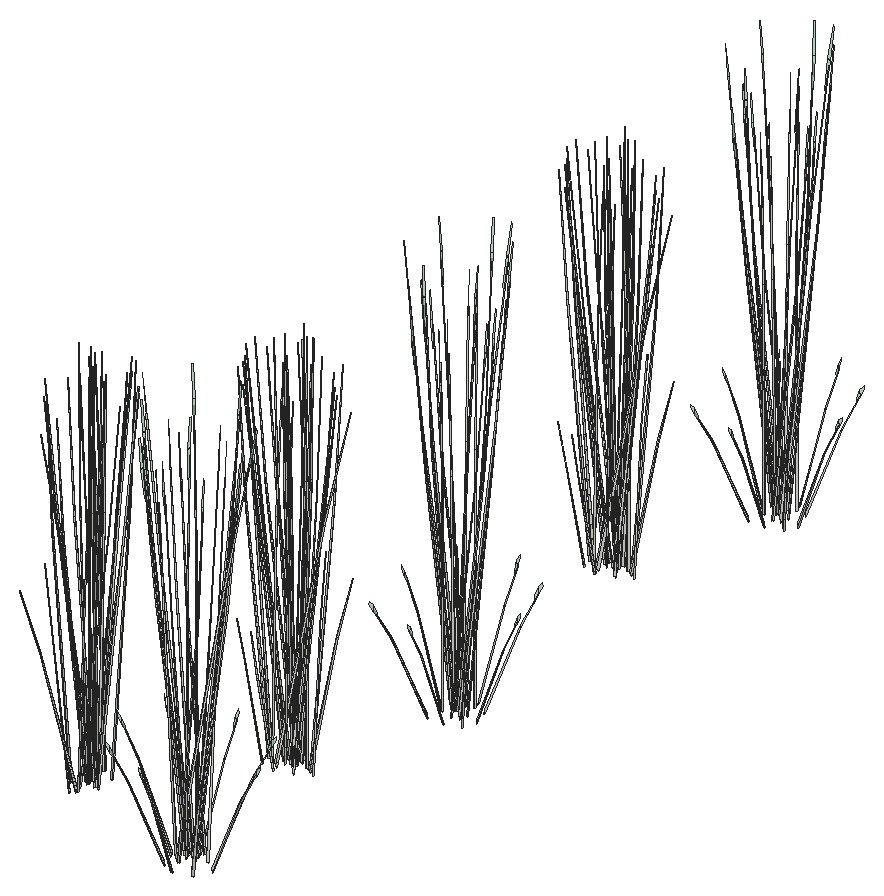
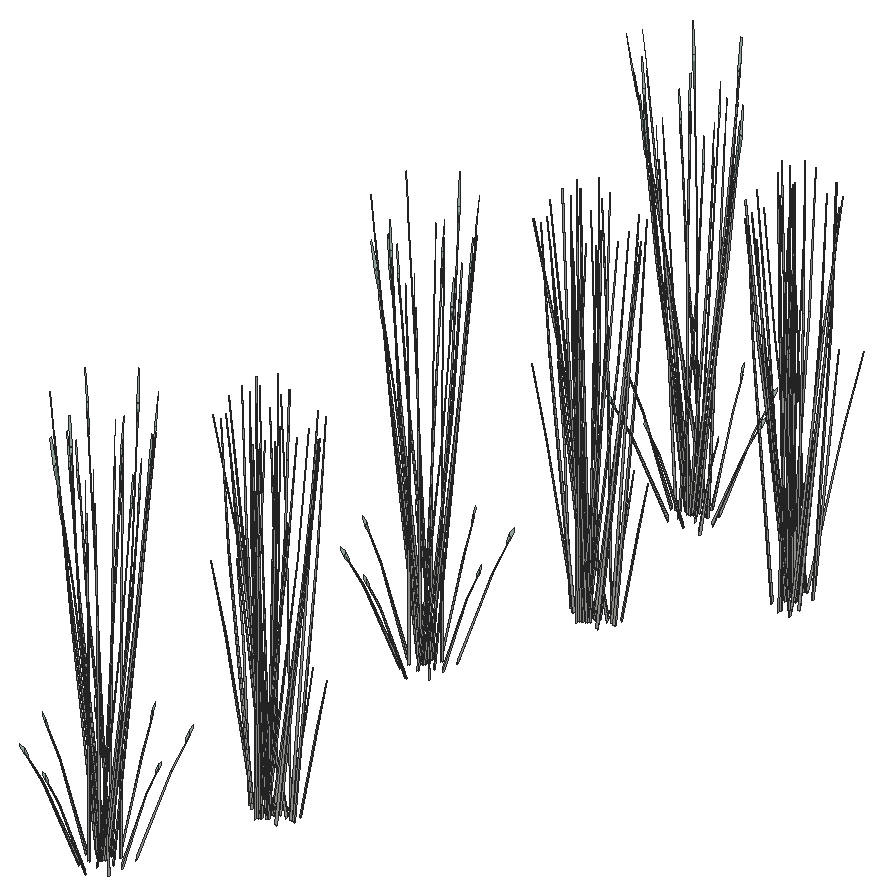
# SketchUp Ruby script. Lengths in inches.
U = 1.inch
M = Sketchup.active_model
def pt(a) = Geom::Point3d.new(a.map { |v| v * U })
def face(e, loops, mat)
  f = e.add_face(loops[0].map { |a| pt(a) })
  loops[1..].each { |l| e.add_face(l.map { |a| pt(a) }).erase! }
  f.material = f.back_material = mat if mat
  f
end
# faces: each face lists its corners as indices into pts; further lists are holes
def faces(e, pts, list, mat = nil) = list.each { |f| face(e, (f[0].is_a?(Array) ? f : [f]).map { |l| l.map { |i| pts[i] } }, mat) }
# xy, xz, yz: faces in a plane at the given z, y or x. An outline is a flat list of corners, or four numbers for a rectangle; further outlines are holes
def ring(l) = l.size == 4 ? [[l[0], l[1]], [l[2], l[1]], [l[2], l[3]], [l[0], l[3]]] : l.each_slice(2).to_a
def flat(e, list, mat, &to3) = list.each { |f| face(e, (f[0].is_a?(Array) ? f : [f]).map { |l| ring(l).map { |u, v| to3.(u, v) } }, mat) }
def xy(e, z, list, mat = nil) = flat(e, list, mat) { |x, y| [x, y, z] }
def xz(e, y, list, mat = nil) = flat(e, list, mat) { |x, z| [x, y, z] }
def yz(e, x, list, mat = nil) = flat(e, list, mat) { |y, z| [x, y, z] }
def lines(e, pts, list) = list.each { |a, b| e.add_line(pt(pts[a]), pt(pts[b])) }
# prism: a flat outline (further loops are holes) pulled along v
def prism(e, loops, v, mat = nil)
  f = face(e, loops, mat); d = Geom::Vector3d.new(v.map { |x| x * U })
  f.pushpull(f.normal.samedirection?(d) ? d.length : -d.length)
end
def box(e, o, s, mat = nil) = prism(e, [[o, [o[0] + s[0], o[1], o[2]], [o[0] + s[0], o[1] + s[1], o[2]], [o[0], o[1] + s[1], o[2]]]], [0, 0, s[2]], mat)
def at(x, y, z, deg = 0) = Geom::Transformation.translation(pt([x, y, z])) * Geom::Transformation.rotation(ORIGIN, Z_AXIS, deg.degrees)
def axes(o, x, y, z) = Geom::Transformation.new([*x, 0, *y, 0, *z, 0, *pt(o).to_a, 1])
def part(name) = M.definitions.add(name)
# library, detail: a bought-in or finely detailed component or shape, given as its bounding box
def library(name, o, s) = part(name).tap { |d| box(d.entities, o, s) }
def detail(e, o, s) = box(e.add_group.entities, o, s)
def put(e, d, t, mat = nil) = e.add_instance(d, t).tap { |i| i.material = mat if mat }
def group(e, t, mat = nil) = e.add_group.tap { |g| g.transformation = t; g.material = mat if mat }.entities
root = M.entities
M.materials.add("LightPink_Translucent").color = [175, 214, 192]
M.materials["LightPink_Translucent"].alpha = 0.75
c1 = part("blade")
p = [[2.15,0.21,22],[0,0.17,0],[0.09,0.45,0],[2.18,0.31,22],[2.29,0.31,22],[0.38,0.45,0],
  [2.48,0.24,33],[2.49,0.24,33],[2.48,0.22,33]]
faces(c1.entities,p,[[0,1,2,3],[4,5,2,3],[6,3,4,7],[8,0,3,6]])
c2 = part("blade with seeds\#1")
put(c2.entities,c1,at(0,0,0))
c3 = part("seeds")
p = [[0.3,-0.1,1.38],[-0.01,-0.03,1.59],[-0.01,-0.03,0.03],[0.14,-0.07,-0.07],[0.29,-0.03,3],[0.15,0.01,3.11]]
faces(c3.entities,p,[[0,1,2,3],[1,0,4,5]],"LightPink_Translucent")
c4 = part("blade with seeds")
put(c4.entities,c1,at(0,0,0))
put(c4.entities,c3,axes([2.4,0.25,30.99],[1.5799,-0.05474,1.17369],[-0.12525,1.92788,0.29478],[-0.07173,-0.02425,1.56792]))
put(root,c2,axes([471.87,244.125,138.66],[-0.38183,0.31082,0],[-0.21294,-0.52,-0.42336],[-0.0485,-0.11843,1.343]))
put(root,c2,axes([471.8,245.15,138.46],[0.31114,0.14341,-0.03193],[-0.09571,0.44138,-0.14479],[-0.05089,0.06702,0.47756]))
put(root,c2,axes([472.92,243.51,138.91],[-0.43479,0.05793,-0.23868],[-0.02629,-0.60335,-0.41019],[-0.05792,-0.10625,1.31016]))
put(root,c2,axes([473.38,243.79,138.91],[-0.18181,0.55986,-0.23868],[-0.38374,-0.26958,-0.41019],[-0.09422,0.01759,1.31016]))
put(root,c2,axes([473.23,245.39,138.66],[0,0.62163,0],[-0.42587,0,-0.42336],[-0.097,0,1.343]))
put(root,c2,axes([473.11,244.91,138.63],[0.32036,0.46241,0.25231],[-0.31699,0.46269,-0.29936],[-0.09098,0.01615,1.35263]))
put(root,c2,axes([473.78,243.65,138.72],[-0.45152,-0.13176,-0.1922],[0.07871,-0.62475,0.4206],[-0.06235,0.10917,1.28336]))
put(root,c2,axes([471.96,241.84,138.67],[-0.38183,-0.31082,0],[0.21294,-0.52,-0.42336],[0.0485,-0.11843,1.343]))
put(root,c2,axes([473.47,240.61,138.34],[0.04573,0.32019,1.16148],[-0.36399,0.05096,0.06648],[-0.05509,-0.22426,0.66092]))
put(root,c2,axes([473.15,240.03,138.57],[-0.24366,0.30821,-0.05322],[-0.22326,-0.33756,-0.24131],[-0.01572,-0.09565,0.79594]))
put(root,c2,axes([473.18,242.86,138.53],[-0.4409,0,0],[0,-0.62163,0],[0,0,1.47217]))
put(root,c2,axes([472.64,244.08,138.02],[0.15256,0.48933,1.05766],[-0.43772,0.15575,0.41096],[0.00728,-0.30048,1.20297]))
put(root,c2,axes([473.52,242.7,138.6],[-0.32797,0.46241,-0.0503],[-0.32817,-0.46269,0],[-0.01145,0.01615,1.4403]))
put(root,c2,axes([472.87,242.82,138.91],[-0.25298,-0.50193,-0.23868],[0.35745,-0.33378,-0.41019],[0.0363,-0.12384,1.31016]))
put(root,c2,axes([473.78,243.38,138.91],[0.25298,0.50193,-0.23868],[-0.35745,0.33378,-0.41019],[-0.0363,0.12384,1.31016]))
put(root,c2,axes([473.28,242.44,138.53],[0,-0.5562,0],[0.39449,0,0],[0,0,1.46356]))
put(root,c2,axes([474.2,243.12,138.53],[-0.32851,0.1622,0],[-0.11504,-0.46318,0],[0,0,1.26638]))
put(root,c2,axes([473.45,242.45,138.53],[0.24613,-0.34702,0],[0.24613,0.34702,0],[0,0,1.38858]))
put(root,c2,axes([474.15,242.51,138.51],[-0.12929,-0.52192,-0.15749],[0.37242,-0.1834,0.00007],[-0.01429,-0.05761,1.42656]))
put(root,c2,axes([473.89,242.8125,138.74],[-0.30669,0.48544,-0.20666],[-0.34439,-0.40848,0.45226],[0.03588,0.13072,1.37996]))
put(root,c2,axes([474.35,243.23,138.52],[-0.17107,0.50118,0],[-0.35546,-0.2412,0],[0,0,1.33477]))
put(root,c2,axes([473.36,242.54,138.6],[0.44068,0,-0.04624],[0,0.62163,0],[0.01385,0,1.47144]))
put(root,c2,axes([474.68,244.36,138.66],[0.38183,0.31082,0],[-0.21294,0.52,-0.42336],[-0.0485,0.11843,1.343]))
put(root,c2,axes([474.35,242.66,138.53],[0.17107,-0.50118,0],[0.35546,0.2412,0],[0,0,1.43523]))
put(root,c2,axes([474.73,242.46,138.52],[-0.38316,0.30694,-0.04218],[-0.21294,-0.52,0.42336],[0.03648,0.12814,1.34234]))
put(root,c2,axes([474.21,242.84,138.6],[0.43775,-0.21614,-0.04932],[0.15339,0.61757,0],[0.01529,-0.00755,1.41242]))
put(root,c2,axes([473.64,241.06,138.52],[-0.00305,0.62132,-0.04082],[-0.42587,0,0.4097],[0.09695,0.01953,1.29904]))
put(root,c2,axes([473.42,240.81,138.67],[0,-0.62163,0],[0.42587,0,-0.42336],[0.097,0,1.343]))
put(root,c2,axes([473.27,242.4,138.91],[0.18181,-0.55986,-0.23868],[0.38374,0.26958,-0.41019],[0.09422,-0.01759,1.31016]))
put(root,c2,axes([473.72,242.68,138.91],[0.43479,-0.05793,-0.23868],[0.02629,0.60335,-0.41019],[0.05792,0.10625,1.31016]))
put(root,c2,axes([474.54,242.45,138.63],[0.12385,-0.62237,0.25231],[0.4427,0.1557,-0.29936],[0.05541,0.10301,1.35263]))
put(root,c2,axes([474.78,242.07,138.66],[0.38183,-0.31082,0],[0.21294,0.52,-0.42336],[0.0485,0.11843,1.343]))
put(root,c2,axes([485.02,259.16,138.66],[-0.31082,0.38183,0],[-0.52,-0.21294,-0.42336],[-0.11843,-0.0485,1.343]))
put(root,c2,axes([485.02,309.15,138.66],[-0.31082,0.38183,0],[-0.52,-0.21294,-0.42336],[-0.11843,-0.0485,1.343]))
put(root,c2,axes([484.23,256.28,138.46],[-0.14341,0.31114,-0.03193],[-0.44138,-0.09571,-0.14479],[-0.06702,-0.05089,0.47756]))
put(root,c2,axes([484.23,306.27,138.46],[-0.14341,0.31114,-0.03193],[-0.44138,-0.09571,-0.14479],[-0.06702,-0.05089,0.47756]))
put(root,c2,axes([483.99,257.7,138.66],[-0.62163,0,0],[0,-0.42587,-0.42336],[0,-0.097,1.343]))
put(root,c2,axes([483.99,307.69,138.66],[-0.62163,0,0],[0,-0.42587,-0.42336],[0,-0.097,1.343]))
put(root,c2,axes([486,258.26,138.91],[-0.50193,0.25298,-0.23868],[-0.33378,-0.35745,-0.41019],[-0.12384,-0.0363,1.31016]))
put(root,c2,axes([486,308.24,138.91],[-0.50193,0.25298,-0.23868],[-0.33378,-0.35745,-0.41019],[-0.12384,-0.0363,1.31016]))
put(root,c2,axes([484.47,257.59,138.63],[-0.46241,0.32036,0.25231],[-0.46269,-0.31699,-0.29936],[-0.01615,-0.09098,1.35263]))
put(root,c2,axes([484.47,307.58,138.63],[-0.46241,0.32036,0.25231],[-0.46269,-0.31699,-0.29936],[-0.01615,-0.09098,1.35263]))
put(root,c2,axes([486.5625,258.37,138.74],[-0.48544,-0.30669,-0.20666],[0.40848,-0.34439,0.45226],[-0.13072,0.03588,1.37996]))
put(root,c2,axes([486.5625,308.36,138.74],[-0.48544,-0.30669,-0.20666],[0.40848,-0.34439,0.45226],[-0.13072,0.03588,1.37996]))
put(root,c2,axes([485.72,258.26,138.72],[0.13176,-0.45152,-0.1922],[0.62475,0.07871,0.4206],[-0.10917,-0.06235,1.28336]))
put(root,c2,axes([485.72,308.25,138.72],[0.13176,-0.45152,-0.1922],[0.62475,0.07871,0.4206],[-0.10917,-0.06235,1.28336]))
put(root,c2,axes([486.91,259.21,138.52],[-0.30694,-0.38316,-0.04218],[0.52,-0.21294,0.42336],[-0.12814,0.03648,1.34234]))
put(root,c2,axes([486.91,309.2,138.52],[-0.30694,-0.38316,-0.04218],[0.52,-0.21294,0.42336],[-0.12814,0.03648,1.34234]))
put(root,c2,axes([485.58,257.86,138.91],[-0.55986,-0.18181,-0.23868],[0.26958,-0.38374,-0.41019],[-0.01759,-0.09422,1.31016]))
put(root,c2,axes([485.58,307.84,138.91],[-0.55986,-0.18181,-0.23868],[0.26958,-0.38374,-0.41019],[-0.01759,-0.09422,1.31016]))
put(root,c2,axes([486.69,258.2,138.91],[0.05793,0.43479,-0.23868],[-0.60335,0.02629,-0.41019],[-0.10625,0.05792,1.31016]))
put(root,c2,axes([486.69,308.1875,138.91],[0.05793,0.43479,-0.23868],[-0.60335,0.02629,-0.41019],[-0.10625,0.05792,1.31016]))
put(root,c2,axes([485.93,255.89,138.46],[-0.34354,0.2186,-0.03193],[-0.31478,-0.23941,-0.14479],[-0.02216,-0.06784,0.47756]))
put(root,c2,axes([485.93,305.875,138.46],[-0.34354,0.2186,-0.03193],[-0.31478,-0.23941,-0.14479],[-0.02216,-0.06784,0.47756]))
put(root,c4,axes([488.74,236.22,138.53],[0.01212,0.07018,1.60472],[-0.24435,0.36652,-0.24515],[-0.17356,-0.01847,0.27334]))
put(root,c2,axes([487.3,259.25,138.66],[0.31082,0.38183,0],[-0.52,0.21294,-0.42336],[-0.11843,0.0485,1.343]))
put(root,c2,axes([487.3,309.24,138.66],[0.31082,0.38183,0],[-0.52,0.21294,-0.42336],[-0.11843,0.0485,1.343]))
put(root,c2,axes([486.15,258.83,138.52],[-0.50118,-0.17107,0],[0.2412,-0.35546,0],[0,0,1.33477]))
put(root,c2,axes([486.15,308.8125,138.52],[-0.50118,-0.17107,0],[0.2412,-0.35546,0],[0,0,1.33477]))
put(root,c2,axes([486.93,259.02,138.63],[0.62237,0.12385,0.25231],[-0.1557,0.4427,-0.29936],[-0.10301,0.05541,1.35263]))
put(root,c2,axes([486.93,309,138.63],[0.62237,0.12385,0.25231],[-0.1557,0.4427,-0.29936],[-0.10301,0.05541,1.35263]))
put(root,c2,axes([486.67,258,138.6],[-0.46241,-0.32797,-0.0503],[0.46269,-0.32817,0],[-0.01615,-0.01145,1.4403]))
put(root,c2,axes([486.67,307.99,138.6],[-0.46241,-0.32797,-0.0503],[0.46269,-0.32817,0],[-0.01615,-0.01145,1.4403]))
put(root,c4,axes([488.61,238.1875,138.53],[0.06411,0.04449,1.60472],[0.1087,0.41223,-0.24515],[-0.14209,0.08791,0.27334]))
put(root,c2,axes([486.26,258.68,138.53],[-0.1622,-0.32851,0],[0.46318,-0.11504,0],[0,0,1.26638]))
put(root,c2,axes([486.26,308.67,138.53],[-0.1622,-0.32851,0],[0.46318,-0.11504,0],[0,0,1.26638]))
put(root,c2,axes([486.83,257.84,138.6],[0,0.44068,-0.04624],[-0.62163,0,0],[0,0.01385,1.47144]))
put(root,c2,axes([486.83,307.82,138.6],[0,0.44068,-0.04624],[-0.62163,0,0],[0,0.01385,1.47144]))
put(root,c2,axes([486.52,257.66,138.53],[0,-0.44089,0],[0.62163,0,0],[0,0,1.47217]))
put(root,c2,axes([486.52,307.65,138.53],[0,-0.44089,0],[0.62163,0,0],[0,0,1.47217]))
put(root,c2,axes([486.53,258.69,138.6],[0.21614,0.43775,-0.04932],[-0.61757,0.15339,0],[0.00755,0.01529,1.41242]))
put(root,c2,axes([486.53,308.68,138.6],[0.21614,0.43775,-0.04932],[-0.61757,0.15339,0],[0.00755,0.01529,1.41242]))
put(root,c2,axes([485.25,256.35,138.66],[-0.31082,-0.38183,0],[0.52,-0.21294,-0.42336],[0.11843,-0.0485,1.343]))
put(root,c2,axes([485.25,306.33,138.66],[-0.31082,-0.38183,0],[0.52,-0.21294,-0.42336],[0.11843,-0.0485,1.343]))
put(root,c2,axes([488.32,258.12,138.52],[-0.62132,-0.00305,-0.04082],[0,-0.42587,0.4097],[-0.01953,0.09695,1.29904]))
put(root,c2,axes([488.32,308.1,138.52],[-0.62132,-0.00305,-0.04082],[0,-0.42587,0.4097],[-0.01953,0.09695,1.29904]))
put(root,c2,axes([486.93,257.93,138.53],[0.34702,0.24613,0],[-0.34702,0.24613,0],[0,0,1.38858]))
put(root,c2,axes([486.93,307.92,138.53],[0.34702,0.24613,0],[-0.34702,0.24613,0],[0,0,1.38858]))
put(root,c2,axes([486.71,258.83,138.53],[0.50118,0.17107,0],[-0.2412,0.35546,0],[0,0,1.43523]))
put(root,c2,axes([486.71,308.82,138.53],[0.50118,0.17107,0],[-0.2412,0.35546,0],[0,0,1.43523]))
put(root,c4,axes([489.49,234.4,138.53],[-0.0463,0.05867,1.60472],[-0.46786,0.12648,-0.24515],[-0.11302,-0.11506,0.27334]))
put(root,c2,axes([486.94,257.76,138.53],[0.5562,0,0],[0,0.39448,0],[0,0,1.46356]))
put(root,c2,axes([486.94,307.75,138.53],[0.5562,0,0],[0,0.39448,0],[0,0,1.46356]))
put(root,c2,axes([485.86,257.4,138.91],[-0.05793,-0.43479,-0.23868],[0.60335,-0.02629,-0.41019],[0.10625,-0.05792,1.31016]))
put(root,c2,axes([485.86,307.39,138.91],[-0.05793,-0.43479,-0.23868],[0.60335,-0.02629,-0.41019],[0.10625,-0.05792,1.31016]))
put(root,c2,axes([486.97,257.75,138.91],[0.55986,0.18181,-0.23868],[-0.26958,0.38374,-0.41019],[0.01759,0.09422,1.31016]))
put(root,c2,axes([486.97,307.73,138.91],[0.55986,0.18181,-0.23868],[-0.26958,0.38374,-0.41019],[0.01759,0.09422,1.31016]))
put(root,c4,axes([490.9,236.93,139.6],[-0.48255,0.29566,-0.26477],[-0.32089,-0.41776,-0.45502],[-0.11906,-0.04243,1.45334]))
put(root,c4,axes([489.81,237.55,139.02],[-0.11227,-0.38804,-0.2819],[0.44589,-0.11019,0.2819],[-0.08989,-0.04475,1.26466]))
put(root,c4,axes([491.15,275.0625,138.53],[0.02423,0.07735,1.60472],[-0.13338,0.46528,-0.24515],[-0.15033,0.01361,0.27334]))
put(root,c4,axes([491.15,325.05,138.53],[0.02423,0.07735,1.60472],[-0.13338,0.46528,-0.24515],[-0.15033,0.01361,0.27334]))
put(root,c2,axes([486.87,258.63,138.51],[0.52192,-0.12929,-0.15749],[0.1834,0.37242,0.00007],[0.05761,-0.01429,1.42656]))
put(root,c2,axes([486.87,308.62,138.51],[0.52192,-0.12929,-0.15749],[0.1834,0.37242,0.00007],[0.05761,-0.01429,1.42656]))
put(root,c4,axes([490.59,236.72,139.18],[-0.28711,-0.37379,-0.40713],[0.43489,-0.26322,0.19594],[-0.09291,-0.04625,1.30716]))
put(root,c4,axes([491.2,236.98,139.18],[-0.519,0.02749,-0.40713],[-0.04694,-0.45634,0.19594],[-0.09291,0.04625,1.30716]))
put(root,c2,axes([486.56,257.35,138.91],[0.50193,-0.25298,-0.23868],[0.33378,0.35745,-0.41019],[0.12384,0.0363,1.31016]))
put(root,c2,axes([486.56,307.33,138.91],[0.50193,-0.25298,-0.23868],[0.33378,0.35745,-0.41019],[0.12384,0.0363,1.31016]))
put(root,c2,axes([488.57,257.9,138.67],[0.62163,0,0],[0,0.42587,-0.42336],[0,0.097,1.343]))
put(root,c2,axes([488.57,307.88,138.67],[0.62163,0,0],[0,0.42587,-0.42336],[0,0.097,1.343]))
put(root,c4,axes([491.65,237.99,139.02],[-0.44589,-0.11019,-0.2819],[0.11227,-0.38804,0.2819],[-0.08989,0.04475,1.26466]))
put(root,c4,axes([491.1875,273.09,138.53],[-0.04449,0.06411,1.60472],[-0.41223,0.1087,-0.24515],[-0.08791,-0.14209,0.27334]))
put(root,c4,axes([491.1875,323.07,138.53],[-0.04449,0.06411,1.60472],[-0.41223,0.1087,-0.24515],[-0.08791,-0.14209,0.27334]))
put(root,c4,axes([490.5,236.46,139.6],[-0.53825,-0.21249,-0.26477],[0.25917,-0.44849,-0.45502],[-0.01692,-0.11011,1.45334]))
put(root,c4,axes([491.13,277.11,138.53],[0.06429,0.03482,1.60472],[0.18935,0.43839,-0.24515],[-0.098,0.13291,0.27334]))
put(root,c4,axes([491.13,327.1,138.53],[0.06429,0.03482,1.60472],[0.18935,0.43839,-0.24515],[-0.098,0.13291,0.27334]))
put(root,c2,axes([485.29,257.12,138.02],[-0.48933,0.15256,1.05766],[-0.15575,-0.43772,0.41096],[0.30048,0.00728,1.20297]))
put(root,c2,axes([485.29,307.11,138.02],[-0.48933,0.15256,1.05766],[-0.15575,-0.43772,0.41096],[0.30048,0.00728,1.20297]))
put(root,c4,axes([491.57,236.86,139.6],[0.05569,0.50815,-0.26477],[-0.58006,0.03072,-0.45502],[-0.10214,0.06769,1.45334]))
put(root,c4,axes([489.33,235.95,139.02],[0.33362,-0.27785,-0.2819],[0.33362,0.27785,0.2819],[0,-0.08949,1.26466]))
put(root,c2,axes([487.54,256.44,138.67],[0.31082,-0.38183,0],[0.52,0.21294,-0.42336],[0.11843,0.0485,1.343]))
put(root,c2,axes([487.54,306.43,138.67],[0.31082,-0.38183,0],[0.52,0.21294,-0.42336],[0.11843,0.0485,1.343]))
put(root,c4,axes([492.71,276.26,139.18],[-0.40128,-0.23189,-0.40713],[0.19312,-0.48183,0.19594],[-0.0925,0,1.30716]))
put(root,c4,axes([492.71,326.25,139.18],[-0.40128,-0.23189,-0.40713],[0.19312,-0.48183,0.19594],[-0.0925,0,1.30716]))
put(root,c4,axes([492.51,276.05,139.6],[-0.50815,0.05569,-0.26477],[-0.03072,-0.58006,-0.45502],[-0.06769,-0.10214,1.45334]))
put(root,c4,axes([492.51,326.04,139.6],[-0.50815,0.05569,-0.26477],[-0.03072,-0.58006,-0.45502],[-0.06769,-0.10214,1.45334]))
put(root,c4,axes([492.54,277.49,139.02],[-0.27785,-0.33362,-0.2819],[0.27785,-0.33362,0.2819],[-0.08949,0,1.26466]))
put(root,c4,axes([492.54,327.47,139.02],[-0.27785,-0.33362,-0.2819],[0.27785,-0.33362,0.2819],[-0.08949,0,1.26466]))
put(root,c2,axes([489.35,257.63,138.57],[-0.30821,-0.24366,-0.05322],[0.33756,-0.22326,-0.24131],[0.09565,-0.01572,0.79594]))
put(root,c2,axes([489.35,307.62,138.57],[-0.30821,-0.24366,-0.05322],[0.33756,-0.22326,-0.24131],[0.09565,-0.01572,0.79594]))
put(root,c4,axes([493.05,276.32,139.6],[-0.21249,0.53825,-0.26477],[-0.44849,-0.25917,-0.45502],[-0.11011,0.01692,1.45334]))
put(root,c4,axes([493.05,326.3,139.6],[-0.21249,0.53825,-0.26477],[-0.44849,-0.25917,-0.45502],[-0.11011,0.01692,1.45334]))
put(root,c4,axes([491.39,276.125,139.02],[0.11019,-0.44589,-0.2819],[0.38804,0.11227,0.2819],[-0.04475,-0.08989,1.26466]))
put(root,c4,axes([491.39,326.11,139.02],[0.11019,-0.44589,-0.2819],[0.38804,0.11227,0.2819],[-0.04475,-0.08989,1.26466]))
put(root,c4,axes([490.92,233.84,138.53],[-0.08017,0.01605,1.60472],[-0.44332,-0.18061,-0.24515],[0.00744,-0.15065,0.27334]))
put(root,c4,axes([490.56,236.125,139.18],[0.23189,-0.40128,-0.40713],[0.48183,0.19312,0.19594],[0,-0.0925,1.30716]))
put(root,c4,axes([490.58,238.23,138.53],[0.07735,-0.02423,1.60472],[0.46528,0.13338,-0.24515],[0.01361,0.15033,0.27334]))
put(root,c4,axes([491.78,236.66,139.18],[-0.23189,0.40128,-0.40713],[-0.48183,-0.19312,0.19594],[0,0.0925,1.30716]))
put(root,c4,axes([492.39,275.68,139.18],[-0.02749,-0.519,-0.40713],[0.45634,-0.04694,0.19594],[-0.04625,-0.09291,1.30716]))
put(root,c4,axes([492.39,325.67,139.18],[-0.02749,-0.519,-0.40713],[0.45634,-0.04694,0.19594],[-0.04625,-0.09291,1.30716]))
put(root,c4,axes([493.3,276.22,139.18],[-0.37379,0.28711,-0.40713],[-0.26322,-0.43489,0.19594],[-0.04625,0.09291,1.30716]))
put(root,c4,axes([493.3,326.21,139.18],[-0.37379,0.28711,-0.40713],[-0.26322,-0.43489,0.19594],[-0.04625,0.09291,1.30716]))
put(root,c2,axes([488.76,257.95,138.34],[-0.32019,0.04573,1.16148],[-0.05096,-0.36399,0.06648],[0.22426,-0.05509,0.66092]))
put(root,c2,axes([488.76,307.94,138.34],[-0.32019,0.04573,1.16148],[-0.05096,-0.36399,0.06648],[0.22426,-0.05509,0.66092]))
put(root,c4,axes([493.01,236.83,139.02],[-0.33362,0.27785,-0.2819],[-0.33362,-0.27785,0.2819],[0,0.08949,1.26466]))
put(root,c4,axes([490.77,235.93,139.6],[-0.05569,-0.50815,-0.26477],[0.58006,-0.03072,-0.45502],[0.10214,-0.06769,1.45334]))
put(root,c4,axes([494.13,277.01,139.02],[-0.38804,0.11227,-0.2819],[-0.11019,-0.44589,0.2819],[-0.04475,0.08989,1.26466]))
put(root,c4,axes([494.13,327,139.02],[-0.38804,0.11227,-0.2819],[-0.11019,-0.44589,0.2819],[-0.04475,0.08989,1.26466]))
put(root,c4,axes([491.84,236.33,139.6],[0.53825,0.21249,-0.26477],[-0.25917,0.44849,-0.45502],[0.01692,0.11011,1.45334]))
put(root,c4,axes([492.45,275.38,139.6],[-0.29566,-0.48255,-0.26477],[0.41776,-0.32089,-0.45502],[0.04243,-0.11906,1.45334]))
put(root,c4,axes([492.45,325.37,139.6],[-0.29566,-0.48255,-0.26477],[0.41776,-0.32089,-0.45502],[0.04243,-0.11906,1.45334]))
put(root,c4,axes([490.69,234.8,139.02],[0.44589,0.11019,-0.2819],[-0.11227,0.38804,0.2819],[0.08989,-0.04475,1.26466]))
put(root,c4,axes([493.51,275.92,139.6],[0.29566,0.48255,-0.26477],[-0.41776,0.32089,-0.45502],[-0.04243,0.11906,1.45334]))
put(root,c4,axes([493.51,325.9,139.6],[0.29566,0.48255,-0.26477],[-0.41776,0.32089,-0.45502],[-0.04243,0.11906,1.45334]))
put(root,c4,axes([491.83,274.29,139.02],[0.38804,-0.11227,-0.2819],[0.11019,0.44589,0.2819],[0.04475,-0.08989,1.26466]))
put(root,c4,axes([491.83,324.27,139.02],[0.38804,-0.11227,-0.2819],[0.11019,0.44589,0.2819],[0.04475,-0.08989,1.26466]))
put(root,c4,axes([493.15,273.22,138.53],[-0.07018,0.01212,1.60472],[-0.36652,-0.24435,-0.24515],[0.01847,-0.17356,0.27334]))
put(root,c4,axes([493.15,323.2,138.53],[-0.07018,0.01212,1.60472],[-0.36652,-0.24435,-0.24515],[0.01847,-0.17356,0.27334]))
put(root,c4,axes([493.08,278.375,138.53],[0.06761,-0.02498,1.60472],[0.39549,0.17324,-0.24515],[0.00569,0.17476,0.27334]))
put(root,c4,axes([493.08,328.36,138.53],[0.06761,-0.02498,1.60472],[0.39549,0.17324,-0.24515],[0.00569,0.17476,0.27334]))
put(root,c4,axes([493.78,274.7,138.62],[-0.17829,-0.47044,1.17325],[0.51157,-0.14973,0.45588],[-0.00851,0.28888,1.33444]))
put(root,c4,axes([493.78,324.6875,138.62],[-0.17829,-0.47044,1.17325],[0.51157,-0.14973,0.45588],[-0.00851,0.28888,1.33444]))
put(root,c4,axes([491.74,236.07,139.18],[0.28711,0.37379,-0.40713],[-0.43489,0.26322,0.19594],[0.09291,0.04625,1.30716]))
put(root,c4,axes([492.66,275.07,139.18],[0.37379,-0.28711,-0.40713],[0.26322,0.43489,0.19594],[0.04625,-0.09291,1.30716]))
put(root,c4,axes([492.66,325.06,139.18],[0.37379,-0.28711,-0.40713],[0.26322,0.43489,0.19594],[0.04625,-0.09291,1.30716]))
put(root,c4,axes([492.53,235.24,139.02],[0.11227,0.38804,-0.2819],[-0.44589,0.11019,0.2819],[0.08989,0.04475,1.26466]))
put(root,c4,axes([491.4375,235.86,139.6],[0.48255,-0.29566,-0.26477],[0.32089,0.41776,-0.45502],[0.11906,0.04243,1.45334]))
put(root,c4,axes([490.22,235.6,138.62],[-0.47044,0.17829,1.17325],[-0.14973,-0.51157,0.45588],[0.28888,0.00851,1.33444]))
put(root,c4,axes([492.88,234.61,138.53],[-0.07154,-0.03508,1.60472],[-0.18375,-0.39195,-0.24515],[0.12396,-0.10636,0.27334]))
put(root,c4,axes([494.57,275.17,139.02],[-0.11019,0.44589,-0.2819],[-0.38804,-0.11227,0.2819],[0.04475,0.08989,1.26466]))
put(root,c4,axes([494.57,325.16,139.02],[-0.11019,0.44589,-0.2819],[-0.38804,-0.11227,0.2819],[0.04475,0.08989,1.26466]))
put(root,c4,axes([492.63,238.24,138.53],[0.03482,-0.06429,1.60472],[0.43839,-0.18935,-0.24515],[0.13291,0.098,0.27334]))
put(root,c4,axes([492.92,274.98,139.6],[0.21249,-0.53825,-0.26477],[0.44849,0.25917,-0.45502],[0.11011,-0.01692,1.45334]))
put(root,c4,axes([492.92,324.97,139.6],[0.21249,-0.53825,-0.26477],[0.44849,0.25917,-0.45502],[0.11011,-0.01692,1.45334]))
put(root,c4,axes([493.42,273.81,139.02],[0.27785,0.33362,-0.2819],[-0.27785,0.33362,0.2819],[0.08949,0,1.26466]))
put(root,c4,axes([493.42,323.8,139.02],[0.27785,0.33362,-0.2819],[-0.27785,0.33362,0.2819],[0.08949,0,1.26466]))
put(root,c4,axes([493.45,275.25,139.6],[0.50815,-0.05569,-0.26477],[0.03072,0.58006,-0.45502],[0.06769,0.10214,1.45334]))
put(root,c4,axes([493.45,325.24,139.6],[0.50815,-0.05569,-0.26477],[0.03072,0.58006,-0.45502],[0.06769,0.10214,1.45334]))
put(root,c4,axes([493.25,275.04,139.18],[0.40128,0.23189,-0.40713],[-0.19312,0.48183,0.19594],[0.0925,0,1.30716]))
put(root,c4,axes([493.25,325.02,139.18],[0.40128,0.23189,-0.40713],[-0.19312,0.48183,0.19594],[0.0925,0,1.30716]))
put(root,c4,axes([494.76,277.36,138.53],[0.03508,-0.07154,1.60472],[0.39195,-0.18375,-0.24515],[0.10636,0.12396,0.27334]))
put(root,c4,axes([494.76,327.35,138.53],[0.03508,-0.07154,1.60472],[0.39195,-0.18375,-0.24515],[0.10636,0.12396,0.27334]))
put(root,c4,axes([494.98,273.97,138.53],[-0.05867,-0.0463,1.60472],[-0.12648,-0.46786,-0.24515],[0.11506,-0.11302,0.27334]))
put(root,c4,axes([494.98,323.95,138.53],[-0.05867,-0.0463,1.60472],[-0.12648,-0.46786,-0.24515],[0.11506,-0.11302,0.27334]))
put(root,c4,axes([493.89,236.29,138.53],[-0.02498,-0.06761,1.60472],[0.17324,-0.39549,-0.24515],[0.17476,-0.00569,0.27334]))
put(root,c4,axes([495.53,275.4,138.53],[-0.01605,-0.08017,1.60472],[0.18061,-0.44332,-0.24515],[0.15065,0.00744,0.27334]))
put(root,c4,axes([495.53,325.39,138.53],[-0.01605,-0.08017,1.60472],[0.18061,-0.44332,-0.24515],[0.15065,0.00744,0.27334]))
